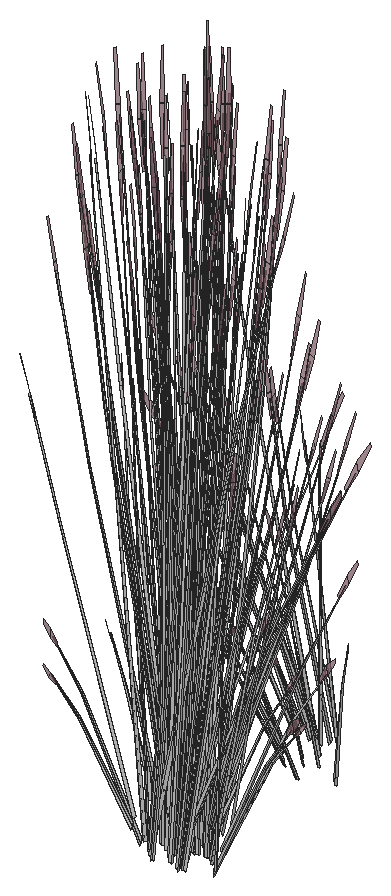
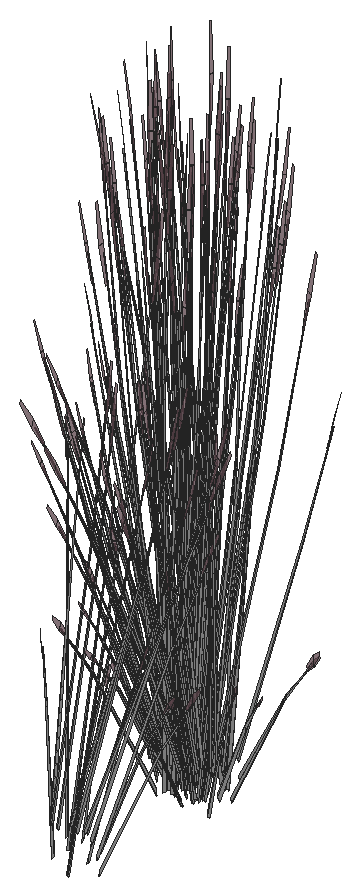
# SketchUp Ruby script. Lengths in inches.
U = 1.inch
M = Sketchup.active_model
def pt(a) = Geom::Point3d.new(a.map { |v| v * U })
def face(e, loops, mat)
  f = e.add_face(loops[0].map { |a| pt(a) })
  loops[1..].each { |l| e.add_face(l.map { |a| pt(a) }).erase! }
  f.material = f.back_material = mat if mat
  f
end
# faces: each face lists its corners as indices into pts; further lists are holes
def faces(e, pts, list, mat = nil) = list.each { |f| face(e, (f[0].is_a?(Array) ? f : [f]).map { |l| l.map { |i| pts[i] } }, mat) }
# xy, xz, yz: faces in a plane at the given z, y or x. An outline is a flat list of corners, or four numbers for a rectangle; further outlines are holes
def ring(l) = l.size == 4 ? [[l[0], l[1]], [l[2], l[1]], [l[2], l[3]], [l[0], l[3]]] : l.each_slice(2).to_a
def flat(e, list, mat, &to3) = list.each { |f| face(e, (f[0].is_a?(Array) ? f : [f]).map { |l| ring(l).map { |u, v| to3.(u, v) } }, mat) }
def xy(e, z, list, mat = nil) = flat(e, list, mat) { |x, y| [x, y, z] }
def xz(e, y, list, mat = nil) = flat(e, list, mat) { |x, z| [x, y, z] }
def yz(e, x, list, mat = nil) = flat(e, list, mat) { |y, z| [x, y, z] }
def lines(e, pts, list) = list.each { |a, b| e.add_line(pt(pts[a]), pt(pts[b])) }
# prism: a flat outline (further loops are holes) pulled along v
def prism(e, loops, v, mat = nil)
  f = face(e, loops, mat); d = Geom::Vector3d.new(v.map { |x| x * U })
  f.pushpull(f.normal.samedirection?(d) ? d.length : -d.length)
end
def box(e, o, s, mat = nil) = prism(e, [[o, [o[0] + s[0], o[1], o[2]], [o[0] + s[0], o[1] + s[1], o[2]], [o[0], o[1] + s[1], o[2]]]], [0, 0, s[2]], mat)
def at(x, y, z, deg = 0) = Geom::Transformation.translation(pt([x, y, z])) * Geom::Transformation.rotation(ORIGIN, Z_AXIS, deg.degrees)
def axes(o, x, y, z) = Geom::Transformation.new([*x, 0, *y, 0, *z, 0, *pt(o).to_a, 1])
def part(name) = M.definitions.add(name)
# library, detail: a bought-in or finely detailed component or shape, given as its bounding box
def library(name, o, s) = part(name).tap { |d| box(d.entities, o, s) }
def detail(e, o, s) = box(e.add_group.entities, o, s)
def put(e, d, t, mat = nil) = e.add_instance(d, t).tap { |i| i.material = mat if mat }
def group(e, t, mat = nil) = e.add_group.tap { |g| g.transformation = t; g.material = mat if mat }.entities
root = M.entities
M.materials.add("LightPink_Translucent").color = [144, 107, 117]
M.materials["LightPink_Translucent"].alpha = 0.75
M.materials.add("[_0053_Ivory_]").color = [200, 200, 200]
c1 = part("blade")
p = [[2.15,0.21,22],[0,0.17,0],[0.09,0.45,0],[2.18,0.31,22],[2.29,0.31,22],[0.38,0.45,0],
  [2.48,0.24,33],[2.49,0.24,33],[2.48,0.22,33]]
faces(c1.entities,p,[[0,1,2,3],[4,5,2,3],[6,3,4,7],[8,0,3,6]])
c2 = part("seeds")
p = [[0.3,-0.1,1.38],[-0.01,-0.03,1.59],[-0.01,-0.03,0.03],[0.14,-0.07,-0.07],[0.29,-0.03,3],[0.15,0.01,3.11]]
faces(c2.entities,p,[[0,1,2,3],[1,0,4,5]],"LightPink_Translucent")
c3 = part("blade with seeds")
put(c3.entities,c1,at(0,0,0))
put(c3.entities,c2,axes([2.4,0.25,30.99],[1.5799,-0.05474,1.17369],[-0.12525,1.92788,0.29478],[-0.07173,-0.02425,1.56792]))
put(root,c3,axes([643.41,186.77,128.68],[0.56663,0.1556,-0.30978],[-0.14267,0.54795,0.30978],[0.11423,-0.06319,1.38974]),"[_0053_Ivory_]")
put(root,c3,axes([641.8,188.67,128.98],[-0.56493,0.5287,0.30756],[-0.56528,-0.52313,-0.36492],[-0.01973,-0.15014,1.64885]),"[_0053_Ivory_]")
put(root,c3,axes([643.6,188.92,129.09],[0.68433,0.30479,0.24065],[-0.32934,0.63331,0.50002],[0,-0.14599,1.60543]),"[_0053_Ivory_]")
put(root,c3,axes([643.33,189.77,129.09],[0.16098,-0.74515,-0.23429],[0.76326,0.12989,0.51271],[-0.13337,-0.1029,1.5644]),"[_0053_Ivory_]")
put(root,c3,axes([641.63,187.58,131.33],[-0.44101,0.41656,-0.51099],[-0.38623,-0.44004,-0.3958],[-0.22407,-0.06338,0.97773]),"[_0053_Ivory_]")
put(root,c3,axes([640.64,188.125,129.42],[0.38775,-0.045,1.1486],[-0.24596,0.39648,0.84392],[-0.19161,-0.05948,0.25299]),"[_0053_Ivory_]")
put(root,c3,axes([643.38,188.49,129.37],[-0.65953,0.03882,0.44739],[-0.05964,-0.64439,-0.21531],[0.11807,-0.06531,1.43643]),"[_0053_Ivory_]")
put(root,c3,axes([641.68,188.96,129.13],[0,0.62885,0.49651],[-0.67951,0,0],[0,-0.14322,1.57504]),"[_0053_Ivory_]")
put(root,c3,axes([646.45,189.1,131.33],[0.16454,-0.57202,-0.51099],[0.56413,0.19607,-0.3958],[0.22713,-0.05245,0.97773]),"[_0053_Ivory_]")
put(root,c3,axes([645.55,186.77,129.03],[0.37973,-0.63014,0],[0.6353,0.35142,-0.51607],[0.14469,0.08004,1.63711]),"[_0053_Ivory_]")
put(root,c3,axes([643.28,189.47,128.86],[-0.36485,-0.52782,-0.44739],[0.55265,-0.37168,0.21531],[-0.11807,-0.06531,1.43643]),"[_0053_Ivory_]")
put(root,c3,axes([643.36,188.73,129.01],[0.26406,0.70318,0.45755],[-0.7545,0.24452,0.17955],[0.00922,-0.12921,1.58856]),"[_0053_Ivory_]")
put(root,c3,axes([647.05,189.27,128.64],[-0.39118,0.07547,1.41583],[-0.06226,-0.6007,0.08104],[0.27398,-0.09092,0.80566]),"[_0053_Ivory_]")
put(root,c3,axes([647.76,188.73,128.91],[-0.37654,-0.40212,-0.06488],[0.4124,-0.36845,-0.29416],[0.11685,-0.02594,0.97024]),"[_0053_Ivory_]")
put(root,c3,axes([643.22,189.28,129.37],[-0.29468,0.56664,0.44739],[-0.61229,-0.27271,-0.21531],[0,-0.13062,1.43643]),"[_0053_Ivory_]")
put(root,c3,axes([644.31,188.79,128.86],[0,-0.72763,0],[0.75945,0,0],[0,0,1.79456]),"[_0053_Ivory_]")
put(root,c3,axes([645.23,187.1,129.13],[-0.56842,-0.31443,0.49651],[0.33976,-0.56381,0],[0.12946,0.07161,1.57504]),"[_0053_Ivory_]")
put(root,c3,axes([646.34,189.3125,131.63],[0.53369,-0.27773,-0.71045],[0.29743,0.5717,0.08574],[0.25786,-0.06494,1.00501]),"[_0053_Ivory_]")
put(root,c3,axes([642.95,189.67,128.71],[-0.63179,-0.1031,-0.62353],[0.13332,-0.63596,-0.16365],[-0.18854,-0.07706,1.37633]),"[_0053_Ivory_]")
put(root,c3,axes([643.95,188.33,129.01],[-0.50358,0.57069,0.45755],[-0.59827,-0.50377,0.17955],[0.1214,-0.05695,1.58856]),"[_0053_Ivory_]")
put(root,c3,axes([644.5,189.35,128.95],[-0.56493,-0.54126,-0.06131],[0.56528,-0.54159,0],[-0.01973,-0.0189,1.75571]),"[_0053_Ivory_]")
put(root,c3,axes([643.07,187.39,129.13],[-0.17545,0.62497,0.17642],[-0.64204,-0.17686,0.35086],[0.11091,-0.00304,1.60407]),"[_0053_Ivory_]")
put(root,c3,axes([642.81,187.89,128.25],[-0.59782,0.25177,1.28929],[-0.19028,-0.72239,0.50096],[0.36709,0.01202,1.46642]),"[_0053_Ivory_]")
put(root,c3,axes([644.41,188.08,129.27],[0.11717,-0.56122,0.1448],[0.57245,0.09742,-0.41347],[0.10418,0.05763,1.26744]),"[_0053_Ivory_]")
put(root,c3,axes([643.42,189.42,129.01],[0.76764,0.13249,0.45755],[-0.15622,0.74829,0.17955],[-0.11218,-0.07226,1.58856]),"[_0053_Ivory_]")
put(root,c3,axes([647.48,188.87,128.15],[-0.03174,-0.09547,1.76342],[0.22015,-0.55846,-0.26939],[0.22208,-0.00803,0.30037]),"[_0053_Ivory_]")
put(root,c3,axes([640.92,188.78,128.15],[0.0154,0.09911,1.76342],[-0.31051,0.51756,-0.26939],[-0.22056,-0.02609,0.30037]),"[_0053_Ivory_]")
put(root,c3,axes([644.17,188.23,129.37],[-0.36485,-0.52782,0.44739],[0.55265,-0.37168,-0.21531],[0.11807,0.06531,1.43643]),"[_0053_Ivory_]")
put(root,c3,axes([642.28,190.64,128.68],[-0.14267,-0.54795,-0.30978],[0.56663,-0.1556,0.30978],[-0.11423,-0.06319,1.38974]),"[_0053_Ivory_]")
put(root,c3,axes([643.01,190.61,129.13],[0.65264,-0.16691,0.17642],[0.16115,0.62115,0.35086],[-0.05821,-0.0905,1.60407]),"[_0053_Ivory_]")
put(root,c3,axes([644.35,188.26,129.32],[0.61322,-0.4175,-0.29095],[0.40778,0.58992,-0.50002],[0.1513,0.05991,1.59708]),"[_0053_Ivory_]")
put(root,c3,axes([646.79,189.36,131.18],[0.50475,0.17543,-0.35414],[-0.14722,0.5118,0.4572],[0.20322,-0.04693,0.87481]),"[_0053_Ivory_]")
put(root,c3,axes([642.125,190.88,128.67],[-0.56842,-0.31443,-0.49651],[0.33976,-0.56381,0],[-0.12946,-0.07161,1.57504]),"[_0053_Ivory_]")
put(root,c3,axes([645.9,187.15,128.67],[0.56842,0.31443,-0.49651],[-0.33976,0.56381,0],[0.12946,0.07161,1.57504]),"[_0053_Ivory_]")
put(root,c3,axes([644.82,188.95,128.86],[0.67951,0,0],[0,0.65103,0],[0,0,1.78407]),"[_0053_Ivory_]")
put(root,c3,axes([643.67,189.77,129.32],[-0.61322,0.4175,-0.29095],[-0.40778,-0.58992,-0.50002],[-0.1513,-0.05991,1.59708]),"[_0053_Ivory_]")
put(root,c3,axes([645.01,187.42,129.13],[-0.65264,0.16691,0.17642],[-0.16115,-0.62115,0.35086],[0.05821,0.0905,1.60407]),"[_0053_Ivory_]")
put(root,c3,axes([645.42,188.73,130.53],[-0.25192,0.01424,1.71376],[0.16712,-0.61729,0.13857],[0.35901,0.03818,0.73262]),"[_0053_Ivory_]")
put(root,c3,axes([645.74,187.39,128.68],[0.14267,0.54795,-0.30978],[-0.56663,0.1556,0.30978],[0.11423,0.06319,1.38974]),"[_0053_Ivory_]")
put(root,c3,axes([644.6,188.62,129.03],[-0.76764,-0.13249,0.49198],[0.15622,-0.74829,0.19306],[0.11218,0.07226,1.70813]),"[_0053_Ivory_]")
put(root,c3,axes([643.99,190.46,128.86],[-0.19817,-0.54216,0],[0.56587,-0.18986,0],[0,0,1.54371]),"[_0053_Ivory_]")
put(root,c3,axes([643.61,189.95,129.27],[-0.11717,0.56122,0.1448],[-0.57245,-0.09742,-0.41347],[-0.10418,-0.05763,1.26744]),"[_0053_Ivory_]")
put(root,c3,axes([644.73,190.39,128.84],[0.63764,-0.21337,-0.19198],[0.22406,0.61462,0.00008],[0.07038,-0.02358,1.73897]),"[_0053_Ivory_]")
put(root,c3,axes([644.95,190.64,129.13],[0.17545,-0.62497,0.17642],[0.64204,0.17686,0.35086],[-0.11091,0.00304,1.60407]),"[_0053_Ivory_]")
put(root,c3,axes([644.81,189.23,128.87],[0.42396,0.40619,0],[-0.42396,0.40619,0],[0,0,1.69266]),"[_0053_Ivory_]")
put(root,c3,axes([645.95,189.05,129.13],[-0.47719,-0.45806,0.17642],[0.48088,-0.44429,0.35086],[-0.0527,0.09355,1.60407]),"[_0053_Ivory_]")
put(root,c3,axes([645.07,188.36,128.71],[0.63179,0.1031,-0.62353],[-0.13332,0.63596,-0.16365],[0.18854,0.07706,1.37633]),"[_0053_Ivory_]")
put(root,c3,axes([647.86,189.47,129.42],[-0.37526,0.10382,1.1486],[0.17664,-0.42906,0.84392],[0.19907,0.02936,0.25299]),"[_0053_Ivory_]")
put(root,c3,axes([643.85,190.71,128.85],[-0.61229,-0.28233,0],[0.29468,-0.58663,0],[0,0,1.62707]),"[_0053_Ivory_]")
put(root,c3,axes([644.36,189.96,129.12],[-0.59306,-0.50614,-0.25192],[0.49904,-0.56836,0.5513],[-0.1597,0.05921,1.68216]),"[_0053_Ivory_]")
put(root,c3,axes([642.8,190.93,129.13],[0.56842,0.31443,0.49651],[-0.33976,0.56381,0],[-0.12946,-0.07161,1.57504]),"[_0053_Ivory_]")
put(root,c3,axes([644.8,188.75,129.37],[0.29468,-0.56664,0.44739],[0.61229,0.27271,-0.21531],[0,0.13062,1.43643]),"[_0053_Ivory_]")
put(root,c3,axes([644.6875,189.08,128.95],[0,0.72727,-0.05637],[-0.75945,0,0],[0,0.02286,1.79368]),"[_0053_Ivory_]")
put(root,c3,axes([644.74,188.5625,128.86],[0.36485,0.52782,-0.44739],[-0.55265,0.37168,0.21531],[0.11807,0.06531,1.43643]),"[_0053_Ivory_]")
put(root,c3,axes([647.21,190.79,130.58],[-0.11624,-0.52862,-0.03492],[0.54943,-0.12153,-0.15832],[0.11473,0.03351,0.52218]),"[_0053_Ivory_]")
put(root,c3,axes([642.47,191.26,129.03],[-0.37973,0.63014,0],[-0.6353,-0.35142,-0.51607],[-0.14469,-0.08004,1.63711]),"[_0053_Ivory_]")
put(root,c3,axes([646.35,189.07,129.13],[0,-0.62885,0.49651],[0.67951,0,0],[0,0.14322,1.57504]),"[_0053_Ivory_]")
put(root,c3,axes([644.65,189.54,129.37],[0.65953,-0.03882,0.44739],[0.05964,0.64439,-0.21531],[-0.11807,0.06531,1.43643]),"[_0053_Ivory_]")
put(root,c3,axes([645.06,188.88,129.27],[0.56587,-0.18339,0.1448],[0.19817,0.52368,-0.41347],[0,0.11525,1.26744]),"[_0053_Ivory_]")
put(root,c3,axes([644.06,189.85,128.86],[-0.65953,0.03882,-0.44739],[-0.05964,-0.64439,0.21531],[-0.11807,0.06531,1.43643]),"[_0053_Ivory_]")
put(root,c3,axes([647.16,190.16,129.24],[-0.14627,-0.15466,1.43002],[0.19032,-0.51164,-0.30754],[0.29594,0.06931,0.61141]),"[_0053_Ivory_]")
put(root,c3,axes([644.55,190.72,128.86],[0.61229,0.28233,0],[-0.29468,0.58663,0],[0,0,1.74954]),"[_0053_Ivory_]")
put(root,c3,axes([644.79,191.34,128.85],[-0.37499,-0.63235,-0.05142],[0.6353,-0.35142,0.51607],[-0.15655,0.0602,1.6363]),"[_0053_Ivory_]")
put(root,c3,axes([644.66,189.82,129.27],[0.44871,0.37783,0.1448],[-0.37428,0.42627,-0.41347],[-0.10418,0.05763,1.26744]),"[_0053_Ivory_]")
put(root,c3,axes([645.82,190.47,131.63],[0.60713,0.01514,-0.71045],[-0.04078,0.63759,0.08574],[0.25721,0.06729,1.00501]),"[_0053_Ivory_]")
put(root,c3,axes([645.13,190.98,129.13],[0.56842,-0.31443,0.49651],[0.33976,0.56381,0],[-0.12946,0.07161,1.57504]),"[_0053_Ivory_]")
put(root,c3,axes([644.32,190.48,128.94],[0.26406,0.72244,-0.06012],[-0.7545,0.25315,0],[0.00922,0.02523,1.72173]),"[_0053_Ivory_]")
put(root,c3,axes([644.62,191.26,128.68],[-0.56663,-0.1556,-0.30978],[0.14267,-0.54795,0.30978],[-0.11423,0.06319,1.38974]),"[_0053_Ivory_]")
put(root,c3,axes([646.81,189.17,129.03],[0.75945,0,0],[0,0.70283,-0.51607],[0,0.16007,1.63711]),"[_0053_Ivory_]")
put(root,c3,axes([646.51,189.54,128.85],[-0.75908,-0.00503,-0.04976],[0,-0.70283,0.49943],[-0.02386,0.16,1.58352]),"[_0053_Ivory_]")
put(root,c3,axes([644.86,188.92,129.32],[0.68399,0.30005,-0.29095],[-0.32934,0.63331,-0.50002],[0.0215,0.15549,1.59708]),"[_0053_Ivory_]")
put(root,c3,axes([640.09,191.26,129.42],[0.25312,-0.28501,1.1486],[0.09988,0.45119,0.84392],[-0.18292,0.08079,0.25299]),"[_0053_Ivory_]")
put(root,c3,axes([646.18,190.73,131.18],[0.34557,0.39372,-0.35414],[-0.39459,0.37271,0.4572],[0.20048,0.05671,0.87481]),"[_0053_Ivory_]")
put(root,c3,axes([646.35,189.64,128.68],[-0.42396,0.39235,-0.30978],[-0.42396,-0.39235,0.30978],[0,0.12637,1.38974]),"[_0053_Ivory_]")
put(root,c3,axes([644.52,189.68,129.32],[0.07077,0.71755,-0.29095],[-0.73712,0.04339,-0.50002],[-0.1298,0.09558,1.59708]),"[_0053_Ivory_]")
put(root,c3,axes([644.79,189.4,128.86],[-0.29468,0.56664,-0.44739],[-0.61229,-0.27271,0.21531],[0,0.13062,1.43643]),"[_0053_Ivory_]")
put(root,c3,axes([641.04,190.03,131.18],[-0.52868,0.08987,-0.35414],[-0.1396,-0.51376,0.4572],[-0.1515,0.13799,0.87481]),"[_0053_Ivory_]")
put(root,c3,axes([644.08,190.22,128.71],[-0.40909,0.47266,-0.62353],[-0.50819,-0.4286,-0.16365],[-0.16393,0.11791,1.37633]),"[_0053_Ivory_]")
put(root,c3,axes([644.81,191.02,128.98],[0.76036,0.2044,0.30756],[-0.19023,0.7306,-0.36492],[-0.12585,0.09144,1.64885]),"[_0053_Ivory_]")
put(root,c3,axes([644.75,191.51,128.67],[-0.56842,0.31443,-0.49651],[-0.33976,-0.56381,0],[-0.12946,0.07161,1.57504]),"[_0053_Ivory_]")
put(root,c3,axes([646.64,189.65,128.67],[0,0.62885,-0.49651],[-0.67951,0,0],[0,0.14322,1.57504]),"[_0053_Ivory_]")
put(root,c3,axes([644.94,189.72,130.53],[-0.2256,-0.10835,1.71376],[0.46687,-0.45453,0.13857],[0.29098,0.20505,0.73262]),"[_0053_Ivory_]")
put(root,c3,axes([645.78,190.96,129.42],[-0.34197,-0.18082,1.1486],[0.44156,-0.18372,0.84392],[0.1191,0.15563,0.25299]),"[_0053_Ivory_]")
put(root,c3,axes([641.96,189.52,130.53],[0.1517,-0.19322,1.71376],[0.38303,0.52154,0.13857],[-0.26271,0.23751,0.73262]),"[_0053_Ivory_]")
put(root,c3,axes([641.48,190.09,131.33],[0.15602,0.5742,-0.51099],[-0.59087,0.10045,-0.3958],[-0.16933,0.15423,0.97773]),"[_0053_Ivory_]")
put(root,c3,axes([645.27,191.42,129.03],[0.37973,0.63014,0],[-0.6353,0.35142,-0.51607],[-0.14469,0.08004,1.63711]),"[_0053_Ivory_]")
put(root,c3,axes([645.87,191.63,128.15],[0.04425,-0.09079,1.76342],[0.55709,-0.26738,-0.26939],[0.16889,0.13839,0.30037]),"[_0053_Ivory_]")
put(root,c3,axes([644.94,188.92,129.5],[-0.01659,-0.59209,1.41272],[0.75089,0.15348,0.59816],[-0.1776,0.32398,1.3335]),"[_0053_Ivory_]")
put(root,c3,axes([645.14,189.57,128.75],[0.2227,0.57576,-0.69212],[-0.64151,0.20736,-0.18165],[0.02462,0.19497,1.52773]),"[_0053_Ivory_]")
put(root,c3,axes([640.76,191.55,128.15],[0.08147,0.06283,1.76342],[0.13814,0.58211,-0.26939],[-0.18056,0.12413,0.30037]),"[_0053_Ivory_]")
put(root,c3,axes([645,191.2,131.33],[0.59932,-0.14948,-0.51099],[0.10484,0.56611,-0.3958],[0.16097,0.16223,0.97773]),"[_0053_Ivory_]")
put(root,c3,axes([645.83,191.78,129.32],[-0.38947,-0.01972,1.0506],[0.25721,-0.41888,0.58006],[0.15386,0.14882,0.8241]),"[_0053_Ivory_]")
put(root,c3,axes([641.84,190,130.53],[0.11309,-0.21615,1.71376],[0.47441,0.44731,0.13857],[-0.21402,0.27879,0.73262]),"[_0053_Ivory_]")
put(root,c3,axes([644.56,190.76,129.24],[0.01072,-0.20846,1.43002],[0.51218,-0.23285,-0.30754],[0.15811,0.2495,0.61141]),"[_0053_Ivory_]")
put(root,c3,axes([641.97,191.21,131.18],[-0.41095,0.33109,-0.35414],[-0.38901,-0.37805,0.4572],[-0.05919,0.19208,0.87481]),"[_0053_Ivory_]")
put(root,c3,axes([642.24,192.5,129.42],[-0.01572,-0.37392,1.1486],[0.39276,0.26669,0.84392],[-0.07724,0.17822,0.25299]),"[_0053_Ivory_]")
put(root,c3,axes([643.27,191.61,128.15],[0.09829,-0.03422,1.76342],[0.59126,0.18834,-0.26939],[0.01729,0.21228,0.30037]),"[_0053_Ivory_]")
put(root,c3,axes([642.38,191.06,131.66],[0.43478,0.42253,-0.5672],[-0.45929,0.37004,-0.43934],[-0.06615,0.21468,1.08528]),"[_0053_Ivory_]")
put(root,c3,axes([641.91,191.69,129.48],[0.55175,-0.11136,0.06507],[0.12684,0.44864,-0.86304],[-0.03498,0.22711,0.7736]),"[_0053_Ivory_]")
put(root,c3,axes([643.67,191.47,131.33],[0.59704,0.15764,-0.51099],[-0.20464,0.54049,-0.3958],[0.05475,0.21761,0.97773]),"[_0053_Ivory_]")
put(root,c3,axes([644.01,190.35,130.53],[-0.13883,-0.2019,1.71376],[0.64153,-0.16998,0.13857],[0.14499,0.31697,0.73262]),"[_0053_Ivory_]")
put(root,c3,axes([643.4,191.8,131.18],[-0.1831,0.48359,-0.35414],[-0.53419,-0.14105,0.4572],[0.04898,0.1947,0.87481]),"[_0053_Ivory_]")
put(root,c3,axes([642.25,190.87,131.99],[-0.0158,0.58168,-0.7886],[-0.66548,-0.03907,0.09517],[-0.07023,0.24643,1.11556]),"[_0053_Ivory_]")
put(root,c3,axes([642.88,190.45,130.53],[-0.01487,-0.24136,1.71376],[0.64429,0.16012,0.13857],[-0.03985,0.34396,0.73262]),"[_0053_Ivory_]")
put(root,c3,axes([643.46,191.37,131.63],[0.28988,0.51132,-0.71045],[-0.59671,0.28496,0.08574],[0.06778,0.24706,1.00501]),"[_0053_Ivory_]")
put(root,c3,axes([641.78,192.17,129.24],[0.19166,-0.0992,1.43002],[0.4732,0.29912,-0.30754],[-0.14084,0.25882,0.61141]),"[_0053_Ivory_]")
put(root,c3,axes([642.03,191.68,130.02],[0.01334,-0.32463,1.54345],[0.60018,0.17147,0.21329],[-0.052,0.34598,0.72882]),"[_0053_Ivory_]")
put(root,c3,axes([642.49,203.99,130.53],[0.13883,0.2019,1.71376],[-0.64153,0.16998,0.13857],[-0.14499,-0.31697,0.73262]),"[_0053_Ivory_]")
put(root,c3,axes([644.98,203.7,129.24],[-0.17264,0.12729,1.43002],[-0.51703,-0.22279,-0.30754],[0.09584,-0.27707,0.61141]),"[_0053_Ivory_]")
put(root,c3,axes([644.2,204.14,131.63],[-0.28988,-0.51132,-0.71045],[0.59671,-0.28496,0.08574],[-0.06778,-0.24706,1.00501]),"[_0053_Ivory_]")
put(root,c3,axes([642.3125,203.46,129.24],[-0.03678,0.20572,1.43002],[-0.53767,0.17221,-0.30754],[-0.12568,-0.26589,0.61141]),"[_0053_Ivory_]")
put(root,c3,axes([643.7,203.01,128.15],[-0.10187,0.02266,1.76342],[-0.56336,-0.25503,-0.26939],[0.00945,-0.21273,0.30037]),"[_0053_Ivory_]")
put(root,c3,axes([645.4,204.64,131.63],[0.0158,-0.58168,-0.71045],[0.66548,0.03907,0.08574],[0.07023,-0.24643,1.00501]),"[_0053_Ivory_]")
put(root,c3,axes([644.25,203.71,131.18],[0.1831,-0.48359,-0.35414],[0.53419,0.14105,0.4572],[-0.04898,-0.1947,0.87481]),"[_0053_Ivory_]")
put(root,c3,axes([644.65,204.35,130.53],[-0.11309,0.21615,1.71376],[-0.47441,-0.44731,0.13857],[0.21402,-0.27879,0.73262]),"[_0053_Ivory_]")
put(root,c3,axes([643.98,204.04,131.33],[-0.59704,-0.15764,-0.51099],[0.20464,-0.54049,-0.3958],[-0.05475,-0.21761,0.97773]),"[_0053_Ivory_]")
put(root,c3,axes([644.35,202.68,129.42],[0.07791,0.3667,1.1486],[-0.43222,-0.2031,0.84392],[0.04651,-0.18776,0.25299]),"[_0053_Ivory_]")
put(root,c3,axes([645.27,204.45,131.33],[-0.43478,-0.42253,-0.51099],[0.45929,-0.37004,-0.3958],[0.06615,-0.21468,0.97773]),"[_0053_Ivory_]")
put(root,c3,axes([645.68,204.29,131.18],[0.41095,-0.33109,-0.35414],[0.38901,0.37805,0.4572],[0.05919,-0.19208,0.87481]),"[_0053_Ivory_]")
put(root,c3,axes([642.125,203.125,129.42],[0.31682,0.21887,1.1486],[-0.4614,0.13157,0.84392],[-0.09872,-0.16821,0.25299]),"[_0053_Ivory_]")
put(root,c3,axes([642.89,204.29,131.63],[-0.51789,-0.30395,-0.71045],[0.36805,-0.53263,0.08574],[-0.18764,-0.18149,1.00501]),"[_0053_Ivory_]")
put(root,c3,axes([642.71,203.88,131.18],[-0.0938,-0.50652,-0.35414],[0.53623,-0.13375,0.4572],[-0.14403,-0.14515,0.87481]),"[_0053_Ivory_]")
put(root,c3,axes([641.875,203.78,128.15],[-0.05883,0.08284,1.76342],[-0.59454,0.17861,-0.26939],[-0.14363,-0.16248,0.30037]),"[_0053_Ivory_]")
put(root,c3,axes([642.86,206.0625,128.75],[-0.24943,-0.64486,-0.69835],[0.71849,-0.23224,-0.18329],[-0.02757,-0.21836,1.54149]),"[_0053_Ivory_]")
put(root,c3,axes([646.19,204.09,128.15],[-0.0909,-0.04954,1.76342],[-0.2335,-0.55347,-0.26939],[0.15752,-0.1502,0.30037]),"[_0053_Ivory_]")
